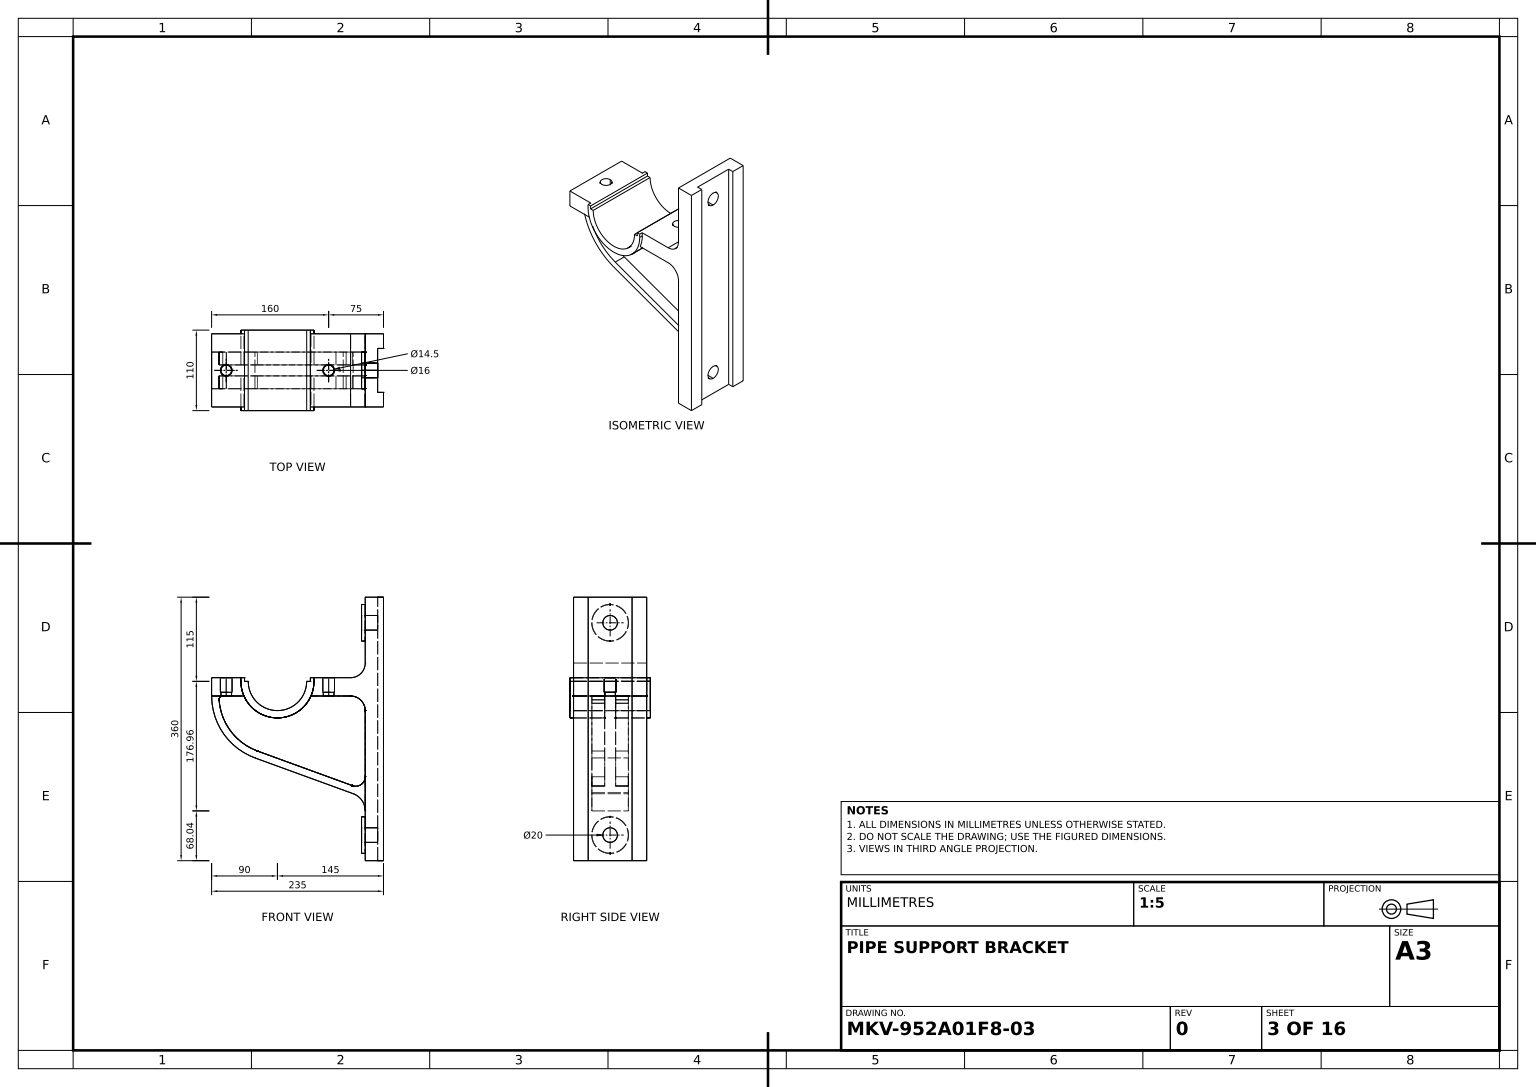
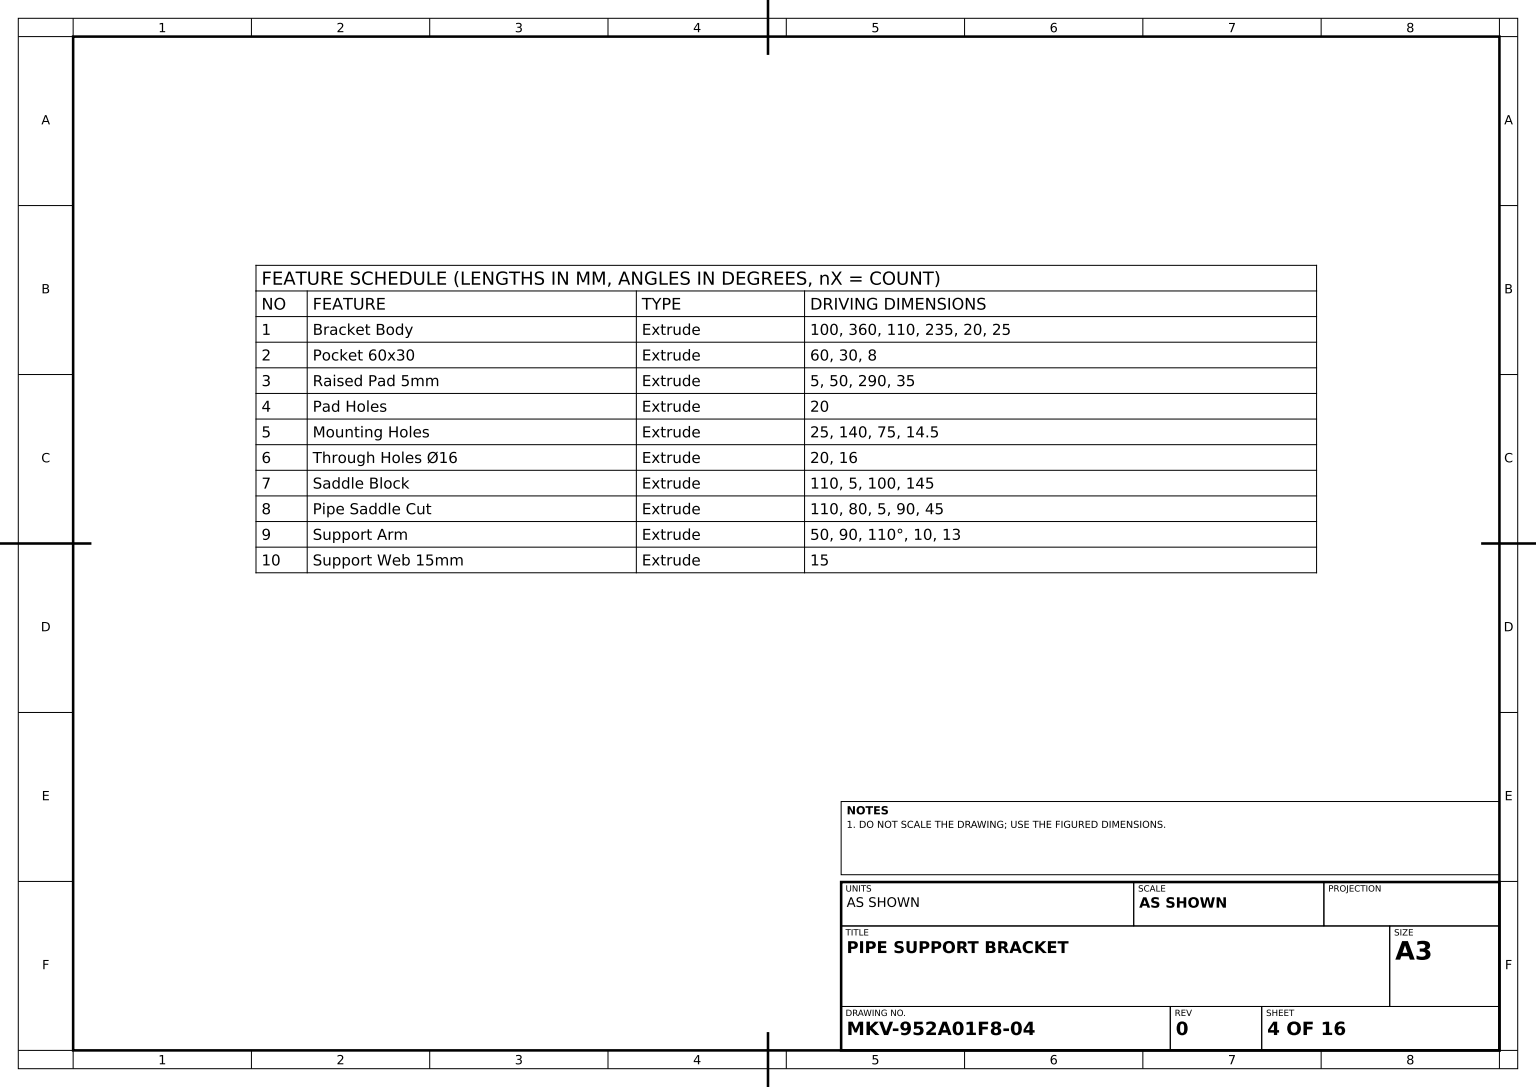
solid
v1 (-41.449496,-158.465301,25)
v2 (-25,-181.957616,25)
e1 v1 v2 CIRCLE(AX(P(-50,-181.957616,25),D(0,0,-1),D(1,0,0)),25)
v3 (-41.449496,-158.465301,-25)
e2 v1 v3 LINE
v4 (-25,-181.957616,-25)
e3 v3 v4 CIRCLE(AX(P(-50,-181.957616,-25),D(0,0,-1),D(1,0,0)),25)
e4 v2 v4 LINE
face CYL(AX(P(-50,-181.957616,25),D(0,0,-1),D(-1,0,0)),25) rev [-e1 e2 e3 -e4]
v5 (-75,0,8)
v6 (-75,0,-8)
e5 v5 v6 CIRCLE(AX(P(-75,0,0),D(0,1,0),D(0,0,1)),8)
v7 (-75,-20,-8)
e6 v7 v6 LINE
v8 (-75,-20,8)
e7 v8 v7 CIRCLE(AX(P(-75,-20,0),D(0,1,0),D(0,0,1)),8)
e8 v8 v5 LINE
face CYL(AX(P(-75,-20,0),D(0,1,0),D(0,0,1)),8) rev [e5 -e6 -e7 e8]
v9 (-172.361611,-100.17541,25)
v10 (-172.361611,-100.17541,7.5)
e9 v9 v10 LINE
v11 (-224.822024,-30.333333,7.5)
e10 v11 v10 CIRCLE(AX(P(-145,-25,7.5),D(0,0,1),D(-1,0,0)),80)
v12 (-224.822024,-30.333333,25)
e11 v12 v11 LINE
e12 v9 v12 CIRCLE(AX(P(-145,-25,25),D(0,0,-1),D(1,0,0)),80)
face CYL(AX(P(-145,-25,25),D(0,0,-1),D(-1,0,0)),80) rev [e9 -e10 -e11 -e12]
v13 (-8,65,0)
v14 (-30,65,0)
e13 v13 v14 LINE
v15 (-30,85,0)
e14 v14 v15 CIRCLE(AX(P(-30,75,0),D(-1,0,0),D(0,-1,0)),10)
v16 (-8,85,0)
e15 v16 v15 LINE
e16 v13 v16 CIRCLE(AX(P(-8,75,0),D(-1,0,0),D(0,0,1)),10)
face CYL(AX(P(0,75,0),D(-1,0,0),D(0,-1,0)),10) rev [e13 e14 -e15 -e16]
v17 (-95,-5,50)
v18 (-99.174243,-25,50)
e17 v17 v18 CIRCLE(AX(P(-145,-5,50),D(0,0,-1),D(1,0,0)),50)
v19 (-45,-25,50)
e18 v18 v19 LINE
v20 (-25,-45,50)
e19 v19 v20 CIRCLE(AX(P(-45,-45,50),D(0,0,-1),D(1,0,0)),20)
v21 (-25,-250,50)
e20 v20 v21 LINE
v22 (0,-250,50)
e21 v21 v22 LINE
v23 (0,110,50)
e22 v22 v23 LINE
v24 (-25,110,50)
e23 v23 v24 LINE
v25 (-25,20,50)
e24 v24 v25 LINE
v26 (-45,0,50)
e25 v25 v26 CIRCLE(AX(P(-45,20,50),D(0,0,-1),D(1,0,0)),20)
v27 (-95.250628,0,50)
e26 v26 v27 LINE
e27 v27 v17 CIRCLE(AX(P(-145,-5,50),D(0,0,-1),D(1,0,0)),50)
face PLANE(AX(P(-45,-45,50),D(0,0,1),D(1,0,0))) [e17 e18 e19 e20 e21 e22 e23 e24 e25 e26 e27]
v28 (-75,-25,-7.25)
v29 (-75,-20,-7.25)
e28 v28 v29 LINE
v30 (-75,-25,7.25)
e29 v30 v28 CIRCLE(AX(P(-75,-25,0),D(0,1,0),D(0,0,1)),7.25)
v31 (-75,-20,7.25)
e30 v30 v31 LINE
e31 v29 v31 CIRCLE(AX(P(-75,-20,0),D(0,-1,0),D(0,0,1)),7.25)
face CYL(AX(P(-75,-25,0),D(0,1,0),D(0,0,1)),7.25) rev [-e28 -e29 e30 -e31]
v32 (0,-250,-50)
v33 (0,110,-50)
e32 v32 v33 LINE
v34 (0,110,-30)
e33 v34 v33 LINE
v35 (0,-250,-30)
e34 v35 v34 LINE
e35 v35 v32 LINE
face PLANE(AX(P(0,110,50),D(-1,0,0),D(0,-1,0))) rev [e32 -e33 -e34 e35]
v36 (-235,-25,25)
v37 (-175.781813,-109.572336,25)
e36 v36 v37 CIRCLE(AX(P(-145,-25,25),D(0,0,1),D(-1,0,0)),90)
e37 v37 v1 LINE
v38 (-25,-135.244726,25)
e38 v2 v38 LINE
v39 (-42.446262,-147.46073,25)
e39 v38 v39 CIRCLE(AX(P(-38,-135.244726,25),D(0,0,-1),D(1,0,0)),13)
e40 v39 v9 LINE
v40 (-224.833148,-30,25)
e41 v12 v40 CIRCLE(AX(P(-219.833148,-30,25),D(0,0,-1),D(1,0,0)),5)
v41 (-219.833148,-25,25)
e42 v40 v41 CIRCLE(AX(P(-219.833148,-30,25),D(0,0,-1),D(1,0,0)),5)
e43 v41 v36 LINE
face PLANE(AX(P(-145,-25,25),D(0,0,-1),D(-1,0,0))) rev [e36 e37 e1 e38 e39 e40 e12 e41 e42 e43]
v42 (-8,110,-30)
e44 v34 v42 LINE
v43 (-8,-250,-30)
e45 v43 v42 LINE
e46 v35 v43 LINE
face PLANE(AX(P(0,-250,-30),D(0,0,-1),D(-1,0,0))) rev [e44 -e45 -e46 e34]
v44 (-195,-5,55)
v45 (-195,-5,50)
e47 v44 v45 LINE
v46 (-194.749372,0,55)
e48 v46 v44 CIRCLE(AX(P(-145,-5,55),D(0,0,1),D(1,0,0)),50)
v47 (-194.749372,0,50)
e49 v46 v47 LINE
e50 v45 v47 CIRCLE(AX(P(-145,-5,50),D(0,0,-1),D(1,0,0)),50)
face CYL(AX(P(-145,-5,55),D(0,0,-1),D(-1,0,0)),50) [-e47 -e48 e49 -e50]
v48 (-100,-5,55)
v49 (-100,0,55)
e51 v48 v49 LINE
v50 (-105,-5,55)
e52 v50 v48 LINE
v51 (-185,-5,55)
e53 v51 v50 CIRCLE(AX(P(-145,-5,55),D(0,0,1),D(1,0,0)),40)
v52 (-190,-5,55)
e54 v52 v51 LINE
v53 (-190,0,55)
e55 v53 v52 LINE
e56 v53 v46 LINE
v54 (-95,-5,55)
e57 v44 v54 CIRCLE(AX(P(-145,-5,55),D(0,0,1),D(1,0,0)),50)
v55 (-95.250628,0,55)
e58 v54 v55 CIRCLE(AX(P(-145,-5,55),D(0,0,1),D(1,0,0)),50)
e59 v55 v49 LINE
face PLANE(AX(P(-145,-5,55),D(0,0,1),D(1,0,0))) [-e51 -e52 -e53 -e54 -e55 e56 e48 e57 e58 e59]
v56 (-8,-225,0)
v57 (-30,-225,0)
e60 v56 v57 LINE
v58 (-8,-205,0)
e61 v58 v56 CIRCLE(AX(P(-8,-215,0),D(-1,0,0),D(0,0,1)),10)
v59 (-30,-205,0)
e62 v58 v59 LINE
e63 v59 v57 CIRCLE(AX(P(-30,-215,0),D(-1,0,0),D(0,-1,0)),10)
face CYL(AX(P(0,-215,0),D(-1,0,0),D(0,-1,0)),10) rev [-e60 -e61 e62 e63]
v60 (-235,-25,-25)
e64 v36 v60 LINE
v61 (-235,-25,50)
e65 v61 v36 LINE
v62 (-235,0,50)
e66 v62 v61 LINE
v63 (-235,0,-50)
e67 v62 v63 LINE
v64 (-235,-25,-50)
e68 v63 v64 LINE
e69 v60 v64 LINE
face PLANE(AX(P(-235,-25,50),D(1,0,0),D(0,0,-1))) rev [-e64 -e65 -e66 e67 e68 -e69]
v65 (-8,110,30)
v66 (0,110,30)
e70 v65 v66 LINE
v67 (0,-250,30)
e71 v67 v66 LINE
v68 (-8,-250,30)
e72 v68 v67 LINE
e73 v68 v65 LINE
face PLANE(AX(P(0,-250,30),D(0,0,1),D(1,0,0))) rev [e70 -e71 -e72 e73]
v69 (-190,-5,-55)
e74 v69 v52 LINE
v70 (-190,0,-55)
e75 v70 v69 LINE
e76 v70 v53 LINE
face PLANE(AX(P(-190,0,-55),D(-1,0,0),D(0,0,1))) rev [-e74 -e75 e76 e55]
e77 v15 v14 CIRCLE(AX(P(-30,75,0),D(-1,0,0),D(0,-1,0)),10)
e78 v16 v13 CIRCLE(AX(P(-8,75,0),D(-1,0,0),D(0,0,1)),10)
face CYL(AX(P(0,75,0),D(-1,0,0),D(0,-1,0)),10) rev [e15 e77 -e13 -e78]
v71 (-175.781813,-109.572336,-25)
e79 v60 v71 CIRCLE(AX(P(-145,-25,-25),D(0,0,1),D(-1,0,0)),90)
e80 v37 v71 LINE
face CYL(AX(P(-145,-25,25),D(0,0,-1),D(-1,0,0)),90) [-e36 e64 e79 -e80]
v72 (-215,-25,7.25)
v73 (-215,-25,-7.25)
e81 v72 v73 CIRCLE(AX(P(-215,-25,0),D(0,1,0),D(0,0,1)),7.25)
e82 v73 v72 CIRCLE(AX(P(-215,-25,0),D(0,1,0),D(0,0,1)),7.25)
face PLANE(AX(P(-219.833148,-25,25),D(0,-1,0),D(1,0,0))) rev [e81 e82]
v74 (-215,-20,8)
v75 (-215,0,8)
e83 v74 v75 LINE
v76 (-215,-20,-8)
e84 v76 v74 CIRCLE(AX(P(-215,-20,0),D(0,1,0),D(0,0,1)),8)
v77 (-215,0,-8)
e85 v76 v77 LINE
e86 v77 v75 CIRCLE(AX(P(-215,0,0),D(0,1,0),D(0,0,1)),8)
face CYL(AX(P(-215,-20,0),D(0,1,0),D(0,0,1)),8) rev [-e83 -e84 e85 e86]
v78 (-25,-45,-7.5)
v79 (-25,-45,-50)
e87 v78 v79 LINE
v80 (-45,-25,-7.5)
e88 v78 v80 CIRCLE(AX(P(-45,-45,-7.5),D(0,0,1),D(1,0,0)),20)
v81 (-45,-25,-50)
e89 v80 v81 LINE
e90 v81 v79 CIRCLE(AX(P(-45,-45,-50),D(0,0,-1),D(1,0,0)),20)
face CYL(AX(P(-45,-45,50),D(0,0,-1),D(-1,0,0)),20) rev [-e87 e88 e89 e90]
v82 (-42.446262,-147.46073,7.5)
e91 v10 v82 LINE
e92 v39 v82 LINE
face PLANE(AX(P(-172.361611,-100.17541,25),D(-0.342020143,-0.939692621,0),D(0.939692621,-0.342020143,0))) rev [-e91 -e9 -e40 e92]
v83 (-215,-20,7.25)
e93 v72 v83 LINE
v84 (-215,-20,-7.25)
e94 v84 v83 CIRCLE(AX(P(-215,-20,0),D(0,-1,0),D(0,0,1)),7.25)
e95 v73 v84 LINE
face CYL(AX(P(-215,-25,0),D(0,1,0),D(0,0,1)),7.25) rev [-e81 e93 -e94 -e95]
v85 (-30,-190,0)
v86 (-30,-240,0)
e96 v85 v86 CIRCLE(AX(P(-30,-215,0),D(-1,0,0),D(0,-1,0)),25)
e97 v86 v85 CIRCLE(AX(P(-30,-215,0),D(-1,0,0),D(0,-1,0)),25)
e98 v57 v59 CIRCLE(AX(P(-30,-215,0),D(-1,0,0),D(0,-1,0)),10)
face PLANE(AX(P(-30,-215,0),D(-1,0,0),D(0,-1,0))) [e96 e97] [-e98 -e63]
v87 (-100,-5,-55)
v88 (-100,0,-55)
e99 v87 v88 LINE
e100 v87 v48 LINE
e101 v88 v49 LINE
face PLANE(AX(P(-100,0,-55),D(1,0,0),D(0,0,-1))) rev [-e99 e100 e51 -e101]
v89 (-99.174243,-25,-50)
v90 (-99.174243,-25,-7.5)
e102 v89 v90 LINE
e103 v89 v81 LINE
e104 v80 v90 LINE
face PLANE(AX(P(-45,-25,50),D(0,1,0),D(-1,0,0))) rev [-e102 e103 -e89 e104]
e105 v31 v29 CIRCLE(AX(P(-75,-20,0),D(0,-1,0),D(0,0,1)),7.25)
e106 v7 v8 CIRCLE(AX(P(-75,-20,0),D(0,1,0),D(0,0,1)),8)
face PLANE(AX(P(-75,-20,0),D(0,1,0),D(0,0,1))) [e31 e105] [e7 e106]
v91 (-25,50,0)
v92 (-25,100,0)
e107 v91 v92 CIRCLE(AX(P(-25,75,0),D(-1,0,0),D(0,1,0)),25)
v93 (-30,100,0)
e108 v93 v92 LINE
v94 (-30,50,0)
e109 v94 v93 CIRCLE(AX(P(-30,75,0),D(-1,0,0),D(0,-1,0)),25)
e110 v94 v91 LINE
face CYL(AX(P(-30,75,0),D(1,0,0),D(0,1,0)),25) [e107 -e108 -e109 e110]
v95 (-25,110,-50)
e111 v33 v95 LINE
e112 v24 v95 LINE
e113 v23 v66 LINE
e114 v42 v65 LINE
face PLANE(AX(P(-25,110,50),D(0,-1,0),D(0,0,-1))) rev [e33 e111 -e112 -e23 e113 -e70 -e114 -e44]
v96 (-219.833148,-25,-7.5)
v97 (-219.833148,-25,-25)
e115 v96 v97 LINE
e116 v97 v60 LINE
v98 (-190.825757,-25,-50)
e117 v64 v98 LINE
v99 (-190.825757,-25,-7.5)
e118 v99 v98 LINE
e119 v99 v96 LINE
face PLANE(AX(P(-45,-25,50),D(0,1,0),D(-1,0,0))) rev [e115 e116 e69 e117 -e118 e119]
e120 v93 v94 CIRCLE(AX(P(-30,75,0),D(-1,0,0),D(0,-1,0)),25)
face PLANE(AX(P(-30,75,0),D(-1,0,0),D(0,-1,0))) [e120 e109] [-e14 -e77]
v100 (-172.361611,-100.17541,-7.5)
v101 (-172.361611,-100.17541,-25)
e121 v100 v101 LINE
v102 (-42.446262,-147.46073,-7.5)
e122 v100 v102 LINE
v103 (-42.446262,-147.46073,-25)
e123 v102 v103 LINE
e124 v103 v101 LINE
face PLANE(AX(P(-172.361611,-100.17541,25),D(-0.342020143,-0.939692621,0),D(0.939692621,-0.342020143,0))) rev [-e121 e122 e123 e124]
e125 v54 v17 LINE
e126 v55 v27 LINE
face CYL(AX(P(-145,-5,55),D(0,0,-1),D(-1,0,0)),50) [-e58 e125 -e27 -e126]
e127 v92 v91 CIRCLE(AX(P(-25,75,0),D(-1,0,0),D(0,1,0)),25)
face CYL(AX(P(-30,75,0),D(1,0,0),D(0,1,0)),25) [-e110 -e120 e108 e127]
e128 v71 v3 LINE
face PLANE(AX(P(-41.449496,-158.465301,25),D(0.342020143,0.939692621,0),D(-0.939692621,0.342020143,0))) rev [e128 -e2 -e37 e80]
v104 (-25,-240,0)
v105 (-25,-190,0)
e129 v104 v105 CIRCLE(AX(P(-25,-215,0),D(-1,0,0),D(0,0,-1)),25)
e130 v85 v105 LINE
e131 v86 v104 LINE
face CYL(AX(P(-30,-215,0),D(1,0,0),D(0,1,0)),25) [e129 -e130 -e97 e131]
v106 (-25,-135.244726,-25)
e132 v4 v106 LINE
v107 (-224.833148,-30,-25)
e133 v107 v97 CIRCLE(AX(P(-219.833148,-30,-25),D(0,0,-1),D(1,0,0)),5)
v108 (-224.822024,-30.333333,-25)
e134 v108 v107 CIRCLE(AX(P(-219.833148,-30,-25),D(0,0,-1),D(1,0,0)),5)
e135 v101 v108 CIRCLE(AX(P(-145,-25,-25),D(0,0,-1),D(1,0,0)),80)
e136 v106 v103 CIRCLE(AX(P(-38,-135.244726,-25),D(0,0,-1),D(1,0,0)),13)
face PLANE(AX(P(-145,-25,-25),D(0,0,-1),D(-1,0,0))) [-e132 -e3 -e128 -e79 -e116 -e133 -e134 -e135 -e124 -e136]
e137 v74 v76 CIRCLE(AX(P(-215,-20,0),D(0,1,0),D(0,0,1)),8)
e138 v75 v77 CIRCLE(AX(P(-215,0,0),D(0,1,0),D(0,0,1)),8)
face CYL(AX(P(-215,-20,0),D(0,1,0),D(0,0,1)),8) rev [-e85 -e137 e83 e138]
v109 (-185,-5,-55)
v110 (-105,-5,-55)
e139 v109 v110 CIRCLE(AX(P(-145,-5,-55),D(0,0,1),D(1,0,0)),40)
e140 v109 v51 LINE
e141 v110 v50 LINE
face CYL(AX(P(-145,-5,-55),D(0,0,1),D(1,0,0)),40) rev [-e139 e140 e53 -e141]
v111 (-99.174243,-25,7.5)
e142 v111 v18 LINE
v112 (-45,-25,7.5)
e143 v112 v111 LINE
e144 v19 v112 LINE
face PLANE(AX(P(-45,-25,50),D(0,1,0),D(-1,0,0))) rev [-e18 -e142 -e143 -e144]
e145 v56 v58 CIRCLE(AX(P(-8,-215,0),D(-1,0,0),D(0,0,1)),10)
face CYL(AX(P(0,-215,0),D(-1,0,0),D(0,-1,0)),10) rev [e60 e98 -e62 -e145]
v113 (-224.822024,-30.333333,-7.5)
e146 v113 v108 LINE
e147 v113 v100 CIRCLE(AX(P(-145,-25,-7.5),D(0,0,1),D(-1,0,0)),80)
face CYL(AX(P(-145,-25,25),D(0,0,-1),D(-1,0,0)),80) rev [e121 e135 -e146 e147]
v114 (-25,-135.244726,-7.5)
e148 v114 v78 LINE
e149 v102 v114 CIRCLE(AX(P(-38,-135.244726,-7.5),D(0,0,1),D(-1,0,0)),13)
v115 (-224.833148,-30,-7.5)
e150 v115 v113 CIRCLE(AX(P(-219.833148,-30,-7.5),D(0,0,1),D(-1,0,0)),5)
e151 v96 v115 CIRCLE(AX(P(-219.833148,-30,-7.5),D(0,0,1),D(-1,0,0)),5)
e152 v90 v99 CIRCLE(AX(P(-145,-5,-7.5),D(0,0,-1),D(1,0,0)),50)
face PLANE(AX(P(-45,-45,-7.5),D(0,0,1),D(1,0,0))) rev [-e148 -e149 -e122 -e147 -e150 -e151 -e119 -e152 -e104 -e88]
v116 (-194.749372,0,-55)
v117 (-195,-5,-55)
e153 v116 v117 CIRCLE(AX(P(-145,-5,-55),D(0,0,1),D(1,0,0)),50)
v118 (-195,-5,-50)
e154 v118 v117 LINE
v119 (-194.749372,0,-50)
e155 v118 v119 CIRCLE(AX(P(-145,-5,-50),D(0,0,-1),D(1,0,0)),50)
e156 v119 v116 LINE
face CYL(AX(P(-145,-5,55),D(0,0,-1),D(-1,0,0)),50) [e153 -e154 e155 e156]
e157 v43 v68 LINE
e158 v22 v67 LINE
v120 (-25,-250,-50)
e159 v21 v120 LINE
e160 v120 v32 LINE
face PLANE(AX(P(0,-250,50),D(0,1,0),D(0,0,1))) rev [e46 e157 e72 -e158 -e21 e159 e160 -e35]
v121 (-219.833148,-25,7.5)
e161 v41 v121 LINE
v122 (-190.825757,-25,7.5)
e162 v122 v121 LINE
v123 (-190.825757,-25,50)
e163 v123 v122 LINE
e164 v61 v123 LINE
face PLANE(AX(P(-45,-25,50),D(0,1,0),D(-1,0,0))) rev [e65 -e43 e161 -e162 -e163 -e164]
v124 (-25,-45,7.5)
e165 v124 v112 CIRCLE(AX(P(-45,-45,7.5),D(0,0,1),D(1,0,0)),20)
e166 v20 v124 LINE
face CYL(AX(P(-45,-45,50),D(0,0,-1),D(-1,0,0)),20) rev [e144 -e165 -e166 -e19]
e167 v6 v5 CIRCLE(AX(P(-75,0,0),D(0,1,0),D(0,0,1)),8)
v125 (-45,0,-50)
e168 v26 v125 LINE
v126 (-95.250628,0,-50)
e169 v125 v126 LINE
v127 (-95.250628,0,-55)
e170 v126 v127 LINE
e171 v127 v88 LINE
face PLANE(AX(P(-235,0,50),D(0,-1,0),D(0,0,-1))) rev [-e167 -e5] [e126 -e26 e168 e169 e170 e171 e101 -e59]
e172 v69 v109 LINE
face PLANE(AX(P(-190,-5,-55),D(0,-1,0),D(1,0,0))) rev [-e172 e74 e54 -e140]
e173 v123 v45 CIRCLE(AX(P(-145,-5,50),D(0,0,-1),D(1,0,0)),50)
e174 v47 v62 LINE
face PLANE(AX(P(-45,-45,50),D(0,0,1),D(1,0,0))) [e164 e173 e50 e174 e66]
v128 (-25,20,-50)
e175 v128 v125 CIRCLE(AX(P(-45,20,-50),D(0,0,-1),D(1,0,0)),20)
e176 v25 v128 LINE
face CYL(AX(P(-45,20,50),D(0,0,-1),D(-1,0,0)),20) rev [e175 -e168 -e25 e176]
e177 v115 v107 LINE
face CYL(AX(P(-219.833148,-30,25),D(0,0,-1),D(-1,0,0)),5) rev [e177 e133 -e115 e151]
e178 v83 v84 CIRCLE(AX(P(-215,-20,0),D(0,-1,0),D(0,0,1)),7.25)
face CYL(AX(P(-215,-25,0),D(0,1,0),D(0,0,1)),7.25) rev [-e82 e95 -e178 -e93]
v129 (-224.833148,-30,7.5)
e179 v40 v129 LINE
e180 v121 v129 CIRCLE(AX(P(-219.833148,-30,7.5),D(0,0,1),D(-1,0,0)),5)
face CYL(AX(P(-219.833148,-30,25),D(0,0,-1),D(-1,0,0)),5) rev [-e42 e179 -e180 -e161]
face CYL(AX(P(-75,-20,0),D(0,1,0),D(0,0,1)),8) rev [-e8 -e106 e6 e167]
face PLANE(AX(P(-215,-20,0),D(0,1,0),D(0,0,1))) [e84 e137] [e94 e178]
v130 (-95,-5,-50)
e181 v126 v130 CIRCLE(AX(P(-145,-5,-50),D(0,0,-1),D(1,0,0)),50)
v131 (-95,-5,-55)
e182 v130 v131 LINE
e183 v131 v127 CIRCLE(AX(P(-145,-5,-55),D(0,0,1),D(1,0,0)),50)
face CYL(AX(P(-145,-5,55),D(0,0,-1),D(-1,0,0)),50) [-e170 e181 e182 e183]
e184 v111 v122 CIRCLE(AX(P(-145,-5,7.5),D(0,0,-1),D(1,0,0)),50)
e185 v129 v11 CIRCLE(AX(P(-219.833148,-30,7.5),D(0,0,1),D(-1,0,0)),5)
v132 (-25,-135.244726,7.5)
e186 v82 v132 CIRCLE(AX(P(-38,-135.244726,7.5),D(0,0,1),D(-1,0,0)),13)
e187 v132 v124 LINE
face PLANE(AX(P(-45,-45,7.5),D(0,0,1),D(1,0,0))) [e165 e143 e184 e162 e180 e185 e10 e91 e186 e187]
face CYL(AX(P(-219.833148,-30,25),D(0,0,-1),D(-1,0,0)),5) rev [e11 -e185 -e179 -e41]
e188 v28 v30 CIRCLE(AX(P(-75,-25,0),D(0,1,0),D(0,0,1)),7.25)
face CYL(AX(P(-75,-25,0),D(0,1,0),D(0,0,1)),7.25) rev [-e105 -e30 -e188 e28]
e189 v105 v104 CIRCLE(AX(P(-25,-215,0),D(-1,0,0),D(0,0,-1)),25)
face CYL(AX(P(-30,-215,0),D(1,0,0),D(0,1,0)),25) [-e96 e130 e189 -e131]
e190 v79 v120 LINE
e191 v38 v132 LINE
e192 v114 v106 LINE
face PLANE(AX(P(-25,-250,50),D(1,0,0),D(0,0,-1))) rev [-e189 -e129] [e148 e87 e190 -e159 -e20 e166 -e187 -e191 -e38 e4 e132 -e192]
face CYL(AX(P(-219.833148,-30,25),D(0,0,-1),D(-1,0,0)),5) rev [e150 e146 e134 -e177]
face PLANE(AX(P(0,110,50),D(-1,0,0),D(0,-1,0))) rev [e158 e71 -e113 -e22]
e193 v98 v118 CIRCLE(AX(P(-145,-5,-50),D(0,0,-1),D(1,0,0)),50)
e194 v119 v63 LINE
face PLANE(AX(P(-45,-45,-50),D(0,0,1),D(1,0,0))) rev [-e193 -e117 -e68 -e194 -e155]
face CYL(AX(P(-145,-5,55),D(0,0,-1),D(-1,0,0)),50) [-e57 e47 -e173 e163 -e184 e142 -e17 -e125]
face PLANE(AX(P(-8,-250,-30),D(-1,0,0),D(0,0,1))) rev [-e73 -e157 e45 e114] [e145 e61] [e78 e16]
face CYL(AX(P(-38,-135.244726,25),D(0,0,-1),D(-1,0,0)),13) rev [e192 e136 -e123 e149]
face CYL(AX(P(-38,-135.244726,25),D(0,0,-1),D(-1,0,0)),13) rev [e191 -e186 -e92 -e39]
e195 v110 v87 LINE
face PLANE(AX(P(-105,-5,-55),D(0,-1,0),D(1,0,0))) rev [-e195 e141 e52 -e100]
e196 v70 v116 LINE
face PLANE(AX(P(-235,0,50),D(0,-1,0),D(0,0,-1))) rev [-e76 e196 -e156 e194 -e67 -e174 -e49 -e56] [-e86 -e138]
e197 v130 v89 CIRCLE(AX(P(-145,-5,-50),D(0,0,-1),D(1,0,0)),50)
e198 v95 v128 LINE
face PLANE(AX(P(-45,-45,-50),D(0,0,1),D(1,0,0))) rev [-e190 -e90 -e103 -e197 -e181 -e169 -e175 -e198 -e111 -e32 -e160]
e199 v117 v131 CIRCLE(AX(P(-145,-5,-55),D(0,0,1),D(1,0,0)),50)
face CYL(AX(P(-145,-5,55),D(0,0,-1),D(-1,0,0)),50) [e154 e199 -e182 e197 e102 e152 e118 e193]
face PLANE(AX(P(-145,-5,-55),D(0,0,1),D(1,0,0))) rev [e75 e172 e139 e195 e99 -e171 -e183 -e199 -e153 -e196]
face PLANE(AX(P(-45,-25,7.5),D(0,-1,0),D(1,0,0))) rev [e188 e29]
face PLANE(AX(P(-25,20,50),D(1,0,0),D(0,1,0))) rev [e198 -e176 -e24 e112] [-e127 -e107]
